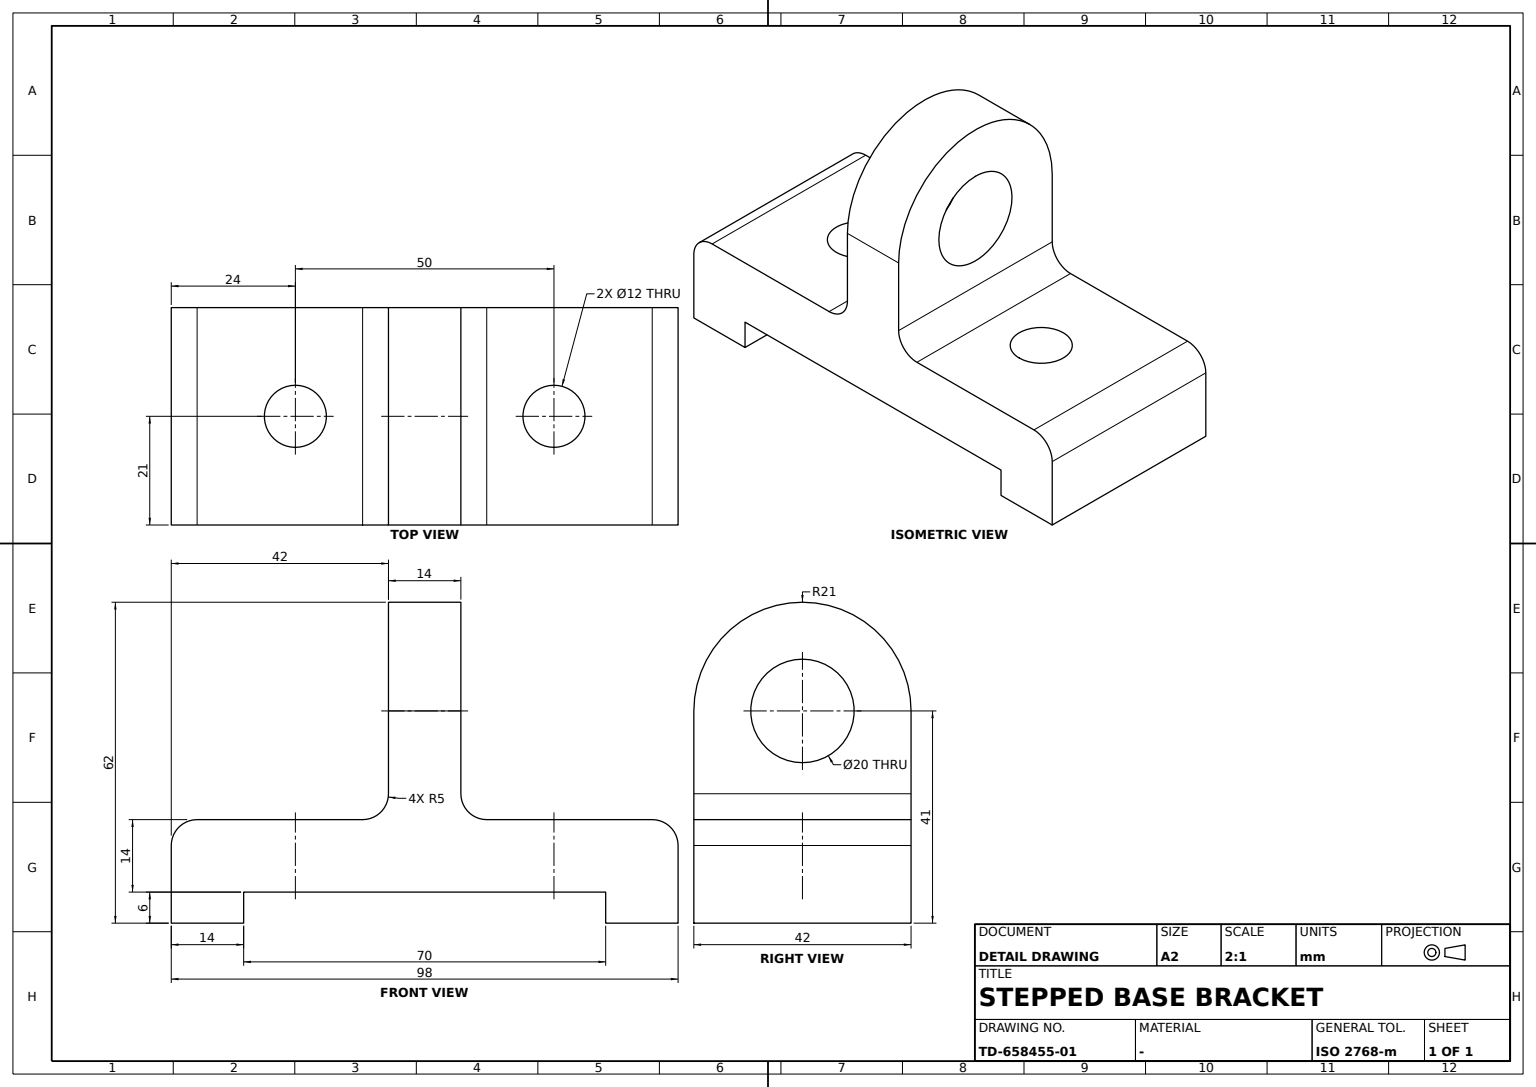
ISO-10303-21;
HEADER;
FILE_DESCRIPTION((''),'2;1');
FILE_NAME('','',(''),(''),'','','');
FILE_SCHEMA(('AUTOMOTIVE_DESIGN'));
ENDSEC;
DATA;
#1=APPLICATION_CONTEXT('');
#2=PRODUCT_CONTEXT('',#1,'mechanical');
#3=PRODUCT('','','',(#2));
#4=PRODUCT_DEFINITION_FORMATION('','',#3);
#5=PRODUCT_DEFINITION_CONTEXT('',#1,'design');
#6=PRODUCT_DEFINITION('','',#4,#5);
#7=PRODUCT_DEFINITION_SHAPE('','',#6);
#8=(LENGTH_UNIT()NAMED_UNIT(*)SI_UNIT(.MILLI.,.METRE.));
#9=(NAMED_UNIT(*)PLANE_ANGLE_UNIT()SI_UNIT($,.RADIAN.));
#10=(NAMED_UNIT(*)SI_UNIT($,.STERADIAN.)SOLID_ANGLE_UNIT());
#11=UNCERTAINTY_MEASURE_WITH_UNIT(LENGTH_MEASURE(0.005),#8,'distance_accuracy_value','');
#12=(GEOMETRIC_REPRESENTATION_CONTEXT(3)GLOBAL_UNCERTAINTY_ASSIGNED_CONTEXT((#11))GLOBAL_UNIT_ASSIGNED_CONTEXT((#8,#9,#10))REPRESENTATION_CONTEXT('',''));
#13=CARTESIAN_POINT('',(-21.,35.,-7.));
#14=VERTEX_POINT('',#13);
#15=CARTESIAN_POINT('',(-21.,35.,-13.));
#16=VERTEX_POINT('',#15);
#17=CARTESIAN_POINT('',(-21.,35.,0.));
#18=DIRECTION('',(0.,0.,-1.));
#19=VECTOR('',#18,1000.);
#20=LINE('',#17,#19);
#21=EDGE_CURVE('',#14,#16,#20,.T.);
#22=ORIENTED_EDGE('',*,*,#21,.T.);
#23=CARTESIAN_POINT('',(21.,35.,-13.));
#24=VERTEX_POINT('',#23);
#25=CARTESIAN_POINT('',(0.,35.,-13.));
#26=DIRECTION('',(1.,0.,0.));
#27=VECTOR('',#26,1000.);
#28=LINE('',#25,#27);
#29=EDGE_CURVE('',#16,#24,#28,.T.);
#30=ORIENTED_EDGE('',*,*,#29,.T.);
#31=CARTESIAN_POINT('',(21.,35.,-7.));
#32=VERTEX_POINT('',#31);
#33=CARTESIAN_POINT('',(21.,35.,0.));
#34=LINE('',#33,#19);
#35=EDGE_CURVE('',#32,#24,#34,.T.);
#36=ORIENTED_EDGE('',*,*,#35,.F.);
#37=CARTESIAN_POINT('',(0.,35.,-7.));
#38=LINE('',#37,#27);
#39=EDGE_CURVE('',#14,#32,#38,.T.);
#40=ORIENTED_EDGE('',*,*,#39,.F.);
#41=EDGE_LOOP('',(#22,#30,#36,#40));
#42=FACE_BOUND('',#41,.T.);
#43=DIRECTION('',(0.,-1.,0.));
#44=AXIS2_PLACEMENT_3D('',#37,#43,#18);
#45=PLANE('',#44);
#46=ADVANCED_FACE('',(#42),#45,.T.);
#47=CARTESIAN_POINT('',(21.,12.,7.));
#48=VERTEX_POINT('',#47);
#49=CARTESIAN_POINT('',(-21.,12.,7.));
#50=VERTEX_POINT('',#49);
#51=CARTESIAN_POINT('',(0.,12.,7.));
#52=DIRECTION('',(-1.,0.,0.));
#53=VECTOR('',#52,1000.);
#54=LINE('',#51,#53);
#55=EDGE_CURVE('',#48,#50,#54,.T.);
#56=ORIENTED_EDGE('',*,*,#55,.T.);
#57=CARTESIAN_POINT('',(-21.,7.,12.));
#58=VERTEX_POINT('',#57);
#59=CARTESIAN_POINT('',(-21.,12.,12.));
#60=AXIS2_PLACEMENT_3D('',#59,#26,#18);
#61=CIRCLE('',#60,5.);
#62=EDGE_CURVE('',#58,#50,#61,.T.);
#63=ORIENTED_EDGE('',*,*,#62,.F.);
#64=CARTESIAN_POINT('',(21.,7.,12.));
#65=VERTEX_POINT('',#64);
#66=CARTESIAN_POINT('',(0.,7.,12.));
#67=LINE('',#66,#53);
#68=EDGE_CURVE('',#65,#58,#67,.T.);
#69=ORIENTED_EDGE('',*,*,#68,.F.);
#70=CARTESIAN_POINT('',(21.,12.,12.));
#71=AXIS2_PLACEMENT_3D('',#70,#26,#18);
#72=CIRCLE('',#71,5.);
#73=EDGE_CURVE('',#65,#48,#72,.T.);
#74=ORIENTED_EDGE('',*,*,#73,.T.);
#75=EDGE_LOOP('',(#56,#63,#69,#74));
#76=FACE_BOUND('',#75,.T.);
#77=CARTESIAN_POINT('',(0.,12.,12.));
#78=AXIS2_PLACEMENT_3D('',#77,#52,#18);
#79=CYLINDRICAL_SURFACE('',#78,5.);
#80=ADVANCED_FACE('',(#76),#79,.F.);
#81=CARTESIAN_POINT('',(-21.,-35.,-7.));
#82=VERTEX_POINT('',#81);
#83=CARTESIAN_POINT('',(21.,-35.,-7.));
#84=VERTEX_POINT('',#83);
#85=CARTESIAN_POINT('',(0.,-35.,-7.));
#86=LINE('',#85,#27);
#87=EDGE_CURVE('',#82,#84,#86,.T.);
#88=ORIENTED_EDGE('',*,*,#87,.T.);
#89=CARTESIAN_POINT('',(21.,-35.,-13.));
#90=VERTEX_POINT('',#89);
#91=CARTESIAN_POINT('',(21.,-35.,0.));
#92=DIRECTION('',(0.,0.,1.));
#93=VECTOR('',#92,1000.);
#94=LINE('',#91,#93);
#95=EDGE_CURVE('',#90,#84,#94,.T.);
#96=ORIENTED_EDGE('',*,*,#95,.F.);
#97=CARTESIAN_POINT('',(-21.,-35.,-13.));
#98=VERTEX_POINT('',#97);
#99=CARTESIAN_POINT('',(0.,-35.,-13.));
#100=LINE('',#99,#27);
#101=EDGE_CURVE('',#98,#90,#100,.T.);
#102=ORIENTED_EDGE('',*,*,#101,.F.);
#103=CARTESIAN_POINT('',(-21.,-35.,0.));
#104=LINE('',#103,#93);
#105=EDGE_CURVE('',#98,#82,#104,.T.);
#106=ORIENTED_EDGE('',*,*,#105,.T.);
#107=EDGE_LOOP('',(#88,#96,#102,#106));
#108=FACE_BOUND('',#107,.T.);
#109=DIRECTION('',(0.,1.,0.));
#110=AXIS2_PLACEMENT_3D('',#99,#109,#92);
#111=PLANE('',#110);
#112=ADVANCED_FACE('',(#108),#111,.T.);
#113=CARTESIAN_POINT('',(-21.,49.,2.));
#114=VERTEX_POINT('',#113);
#115=CARTESIAN_POINT('',(21.,49.,2.));
#116=VERTEX_POINT('',#115);
#117=CARTESIAN_POINT('',(0.,49.,2.));
#118=LINE('',#117,#27);
#119=EDGE_CURVE('',#114,#116,#118,.T.);
#120=ORIENTED_EDGE('',*,*,#119,.F.);
#121=CARTESIAN_POINT('',(-21.,44.,7.));
#122=VERTEX_POINT('',#121);
#123=CARTESIAN_POINT('',(-21.,44.,2.));
#124=AXIS2_PLACEMENT_3D('',#123,#26,#18);
#125=CIRCLE('',#124,5.);
#126=EDGE_CURVE('',#114,#122,#125,.T.);
#127=ORIENTED_EDGE('',*,*,#126,.T.);
#128=CARTESIAN_POINT('',(21.,44.,7.));
#129=VERTEX_POINT('',#128);
#130=CARTESIAN_POINT('',(0.,44.,7.));
#131=LINE('',#130,#27);
#132=EDGE_CURVE('',#122,#129,#131,.T.);
#133=ORIENTED_EDGE('',*,*,#132,.T.);
#134=CARTESIAN_POINT('',(21.,44.,2.));
#135=AXIS2_PLACEMENT_3D('',#134,#26,#18);
#136=CIRCLE('',#135,5.);
#137=EDGE_CURVE('',#116,#129,#136,.T.);
#138=ORIENTED_EDGE('',*,*,#137,.F.);
#139=EDGE_LOOP('',(#120,#127,#133,#138));
#140=FACE_BOUND('',#139,.T.);
#141=CARTESIAN_POINT('',(0.,44.,2.));
#142=AXIS2_PLACEMENT_3D('',#141,#26,#92);
#143=CYLINDRICAL_SURFACE('',#142,5.);
#144=ADVANCED_FACE('',(#140),#143,.T.);
#145=CARTESIAN_POINT('',(-21.,-49.,-13.));
#146=VERTEX_POINT('',#145);
#147=CARTESIAN_POINT('',(-21.,0.,-13.));
#148=VECTOR('',#109,1000.);
#149=LINE('',#147,#148);
#150=EDGE_CURVE('',#146,#98,#149,.T.);
#151=ORIENTED_EDGE('',*,*,#150,.T.);
#152=ORIENTED_EDGE('',*,*,#101,.T.);
#153=CARTESIAN_POINT('',(21.,-49.,-13.));
#154=VERTEX_POINT('',#153);
#155=CARTESIAN_POINT('',(21.,0.,-13.));
#156=LINE('',#155,#148);
#157=EDGE_CURVE('',#154,#90,#156,.T.);
#158=ORIENTED_EDGE('',*,*,#157,.F.);
#159=CARTESIAN_POINT('',(0.,-49.,-13.));
#160=LINE('',#159,#27);
#161=EDGE_CURVE('',#146,#154,#160,.T.);
#162=ORIENTED_EDGE('',*,*,#161,.F.);
#163=EDGE_LOOP('',(#151,#152,#158,#162));
#164=FACE_BOUND('',#163,.T.);
#165=AXIS2_PLACEMENT_3D('',#159,#18,#109);
#166=PLANE('',#165);
#167=ADVANCED_FACE('',(#164),#166,.T.);
#168=CARTESIAN_POINT('',(21.,7.,28.));
#169=VERTEX_POINT('',#168);
#170=CARTESIAN_POINT('',(21.,7.,0.));
#171=LINE('',#170,#19);
#172=EDGE_CURVE('',#169,#65,#171,.T.);
#173=ORIENTED_EDGE('',*,*,#172,.T.);
#174=ORIENTED_EDGE('',*,*,#68,.T.);
#175=CARTESIAN_POINT('',(-21.,7.,28.));
#176=VERTEX_POINT('',#175);
#177=CARTESIAN_POINT('',(-21.,7.,0.));
#178=LINE('',#177,#19);
#179=EDGE_CURVE('',#176,#58,#178,.T.);
#180=ORIENTED_EDGE('',*,*,#179,.F.);
#181=CARTESIAN_POINT('',(0.,7.,28.));
#182=AXIS2_PLACEMENT_3D('',#181,#109,#92);
#183=CIRCLE('',#182,21.);
#184=EDGE_CURVE('',#176,#169,#183,.T.);
#185=ORIENTED_EDGE('',*,*,#184,.T.);
#186=EDGE_LOOP('',(#173,#174,#180,#185));
#187=FACE_BOUND('',#186,.T.);
#188=CARTESIAN_POINT('',(0.,7.,38.));
#189=VERTEX_POINT('',#188);
#190=CIRCLE('',#182,10.);
#191=EDGE_CURVE('',#189,#189,#190,.T.);
#192=ORIENTED_EDGE('',*,*,#191,.F.);
#193=EDGE_LOOP('',(#192));
#194=FACE_BOUND('',#193,.T.);
#195=CARTESIAN_POINT('',(0.,7.,0.));
#196=AXIS2_PLACEMENT_3D('',#195,#109,#52);
#197=PLANE('',#196);
#198=ADVANCED_FACE('',(#187,#194),#197,.T.);
#199=CARTESIAN_POINT('',(-6.,25.,-7.));
#200=VERTEX_POINT('',#199);
#201=CARTESIAN_POINT('',(0.,25.,-7.));
#202=AXIS2_PLACEMENT_3D('',#201,#18,#52);
#203=CIRCLE('',#202,6.);
#204=EDGE_CURVE('',#200,#200,#203,.T.);
#205=ORIENTED_EDGE('',*,*,#204,.T.);
#206=EDGE_LOOP('',(#205));
#207=FACE_BOUND('',#206,.T.);
#208=CARTESIAN_POINT('',(6.,25.,7.));
#209=VERTEX_POINT('',#208);
#210=CARTESIAN_POINT('',(0.,25.,7.));
#211=AXIS2_PLACEMENT_3D('',#210,#92,#26);
#212=CIRCLE('',#211,6.);
#213=EDGE_CURVE('',#209,#209,#212,.T.);
#214=ORIENTED_EDGE('',*,*,#213,.T.);
#215=EDGE_LOOP('',(#214));
#216=FACE_BOUND('',#215,.T.);
#217=CARTESIAN_POINT('',(0.,25.,-3.66));
#218=AXIS2_PLACEMENT_3D('',#217,#92,#109);
#219=CYLINDRICAL_SURFACE('',#218,6.);
#220=ADVANCED_FACE('',(#207,#216),#219,.F.);
#221=CARTESIAN_POINT('',(-6.,-25.,-7.));
#222=VERTEX_POINT('',#221);
#223=CARTESIAN_POINT('',(0.,-25.,-7.));
#224=AXIS2_PLACEMENT_3D('',#223,#18,#52);
#225=CIRCLE('',#224,6.);
#226=EDGE_CURVE('',#222,#222,#225,.T.);
#227=ORIENTED_EDGE('',*,*,#226,.F.);
#228=EDGE_LOOP('',(#227));
#229=FACE_BOUND('',#228,.T.);
#230=ORIENTED_EDGE('',*,*,#204,.F.);
#231=EDGE_LOOP('',(#230));
#232=FACE_BOUND('',#231,.T.);
#233=CARTESIAN_POINT('',(-21.,0.,-7.));
#234=LINE('',#233,#148);
#235=EDGE_CURVE('',#82,#14,#234,.T.);
#236=ORIENTED_EDGE('',*,*,#235,.T.);
#237=ORIENTED_EDGE('',*,*,#39,.T.);
#238=CARTESIAN_POINT('',(21.,0.,-7.));
#239=LINE('',#238,#148);
#240=EDGE_CURVE('',#84,#32,#239,.T.);
#241=ORIENTED_EDGE('',*,*,#240,.F.);
#242=ORIENTED_EDGE('',*,*,#87,.F.);
#243=EDGE_LOOP('',(#236,#237,#241,#242));
#244=FACE_BOUND('',#243,.T.);
#245=AXIS2_PLACEMENT_3D('',#85,#18,#109);
#246=PLANE('',#245);
#247=ADVANCED_FACE('',(#229,#232,#244),#246,.T.);
#248=CARTESIAN_POINT('',(-21.,-44.,7.));
#249=VERTEX_POINT('',#248);
#250=CARTESIAN_POINT('',(-21.,-49.,2.));
#251=VERTEX_POINT('',#250);
#252=CARTESIAN_POINT('',(-21.,-44.,2.));
#253=AXIS2_PLACEMENT_3D('',#252,#26,#18);
#254=CIRCLE('',#253,5.);
#255=EDGE_CURVE('',#249,#251,#254,.T.);
#256=ORIENTED_EDGE('',*,*,#255,.T.);
#257=CARTESIAN_POINT('',(21.,-49.,2.));
#258=VERTEX_POINT('',#257);
#259=CARTESIAN_POINT('',(0.,-49.,2.));
#260=LINE('',#259,#27);
#261=EDGE_CURVE('',#251,#258,#260,.T.);
#262=ORIENTED_EDGE('',*,*,#261,.T.);
#263=CARTESIAN_POINT('',(21.,-44.,7.));
#264=VERTEX_POINT('',#263);
#265=CARTESIAN_POINT('',(21.,-44.,2.));
#266=AXIS2_PLACEMENT_3D('',#265,#26,#18);
#267=CIRCLE('',#266,5.);
#268=EDGE_CURVE('',#264,#258,#267,.T.);
#269=ORIENTED_EDGE('',*,*,#268,.F.);
#270=CARTESIAN_POINT('',(0.,-44.,7.));
#271=LINE('',#270,#27);
#272=EDGE_CURVE('',#249,#264,#271,.T.);
#273=ORIENTED_EDGE('',*,*,#272,.F.);
#274=EDGE_LOOP('',(#256,#262,#269,#273));
#275=FACE_BOUND('',#274,.T.);
#276=CARTESIAN_POINT('',(0.,-44.,2.));
#277=AXIS2_PLACEMENT_3D('',#276,#26,#43);
#278=CYLINDRICAL_SURFACE('',#277,5.);
#279=ADVANCED_FACE('',(#275),#278,.T.);
#280=CARTESIAN_POINT('',(21.,49.,-13.));
#281=VERTEX_POINT('',#280);
#282=EDGE_CURVE('',#24,#281,#156,.T.);
#283=ORIENTED_EDGE('',*,*,#282,.T.);
#284=CARTESIAN_POINT('',(21.,49.,0.));
#285=LINE('',#284,#93);
#286=EDGE_CURVE('',#281,#116,#285,.T.);
#287=ORIENTED_EDGE('',*,*,#286,.T.);
#288=ORIENTED_EDGE('',*,*,#137,.T.);
#289=CARTESIAN_POINT('',(21.,0.,7.));
#290=VECTOR('',#43,1000.);
#291=LINE('',#289,#290);
#292=EDGE_CURVE('',#129,#48,#291,.T.);
#293=ORIENTED_EDGE('',*,*,#292,.T.);
#294=ORIENTED_EDGE('',*,*,#73,.F.);
#295=ORIENTED_EDGE('',*,*,#172,.F.);
#296=CARTESIAN_POINT('',(21.,-7.,28.));
#297=VERTEX_POINT('',#296);
#298=CARTESIAN_POINT('',(21.,0.,28.));
#299=LINE('',#298,#148);
#300=EDGE_CURVE('',#297,#169,#299,.T.);
#301=ORIENTED_EDGE('',*,*,#300,.F.);
#302=CARTESIAN_POINT('',(21.,-7.,12.));
#303=VERTEX_POINT('',#302);
#304=CARTESIAN_POINT('',(21.,-7.,0.));
#305=LINE('',#304,#19);
#306=EDGE_CURVE('',#297,#303,#305,.T.);
#307=ORIENTED_EDGE('',*,*,#306,.T.);
#308=CARTESIAN_POINT('',(21.,-12.,7.));
#309=VERTEX_POINT('',#308);
#310=CARTESIAN_POINT('',(21.,-12.,12.));
#311=AXIS2_PLACEMENT_3D('',#310,#26,#18);
#312=CIRCLE('',#311,5.);
#313=EDGE_CURVE('',#309,#303,#312,.T.);
#314=ORIENTED_EDGE('',*,*,#313,.F.);
#315=EDGE_CURVE('',#309,#264,#291,.T.);
#316=ORIENTED_EDGE('',*,*,#315,.T.);
#317=ORIENTED_EDGE('',*,*,#268,.T.);
#318=CARTESIAN_POINT('',(21.,-49.,0.));
#319=LINE('',#318,#19);
#320=EDGE_CURVE('',#258,#154,#319,.T.);
#321=ORIENTED_EDGE('',*,*,#320,.T.);
#322=ORIENTED_EDGE('',*,*,#157,.T.);
#323=ORIENTED_EDGE('',*,*,#95,.T.);
#324=ORIENTED_EDGE('',*,*,#240,.T.);
#325=ORIENTED_EDGE('',*,*,#35,.T.);
#326=EDGE_LOOP('',(#283,#287,#288,#293,#294,#295,#301,#307,#314,#316,#317,#321,#322,#323,#324,#325));
#327=FACE_BOUND('',#326,.T.);
#328=CARTESIAN_POINT('',(21.,0.,0.));
#329=AXIS2_PLACEMENT_3D('',#328,#26,#109);
#330=PLANE('',#329);
#331=ADVANCED_FACE('',(#327),#330,.T.);
#332=ORIENTED_EDGE('',*,*,#306,.F.);
#333=CARTESIAN_POINT('',(-21.,-7.,28.));
#334=VERTEX_POINT('',#333);
#335=CARTESIAN_POINT('',(0.,-7.,28.));
#336=AXIS2_PLACEMENT_3D('',#335,#109,#92);
#337=CIRCLE('',#336,21.);
#338=EDGE_CURVE('',#334,#297,#337,.T.);
#339=ORIENTED_EDGE('',*,*,#338,.F.);
#340=CARTESIAN_POINT('',(-21.,-7.,12.));
#341=VERTEX_POINT('',#340);
#342=CARTESIAN_POINT('',(-21.,-7.,0.));
#343=LINE('',#342,#19);
#344=EDGE_CURVE('',#334,#341,#343,.T.);
#345=ORIENTED_EDGE('',*,*,#344,.T.);
#346=CARTESIAN_POINT('',(0.,-7.,12.));
#347=LINE('',#346,#27);
#348=EDGE_CURVE('',#341,#303,#347,.T.);
#349=ORIENTED_EDGE('',*,*,#348,.T.);
#350=EDGE_LOOP('',(#332,#339,#345,#349));
#351=FACE_BOUND('',#350,.T.);
#352=CARTESIAN_POINT('',(0.,-7.,38.));
#353=VERTEX_POINT('',#352);
#354=CIRCLE('',#336,10.);
#355=EDGE_CURVE('',#353,#353,#354,.T.);
#356=ORIENTED_EDGE('',*,*,#355,.T.);
#357=EDGE_LOOP('',(#356));
#358=FACE_BOUND('',#357,.T.);
#359=CARTESIAN_POINT('',(0.,-7.,0.));
#360=AXIS2_PLACEMENT_3D('',#359,#109,#52);
#361=PLANE('',#360);
#362=ADVANCED_FACE('',(#351,#358),#361,.F.);
#363=CARTESIAN_POINT('',(-21.,49.,-13.));
#364=VERTEX_POINT('',#363);
#365=EDGE_CURVE('',#16,#364,#149,.T.);
#366=ORIENTED_EDGE('',*,*,#365,.T.);
#367=CARTESIAN_POINT('',(0.,49.,-13.));
#368=LINE('',#367,#27);
#369=EDGE_CURVE('',#364,#281,#368,.T.);
#370=ORIENTED_EDGE('',*,*,#369,.T.);
#371=ORIENTED_EDGE('',*,*,#282,.F.);
#372=ORIENTED_EDGE('',*,*,#29,.F.);
#373=EDGE_LOOP('',(#366,#370,#371,#372));
#374=FACE_BOUND('',#373,.T.);
#375=ADVANCED_FACE('',(#374),#166,.T.);
#376=ORIENTED_EDGE('',*,*,#338,.T.);
#377=ORIENTED_EDGE('',*,*,#300,.T.);
#378=ORIENTED_EDGE('',*,*,#184,.F.);
#379=CARTESIAN_POINT('',(-21.,0.,28.));
#380=LINE('',#379,#148);
#381=EDGE_CURVE('',#334,#176,#380,.T.);
#382=ORIENTED_EDGE('',*,*,#381,.F.);
#383=EDGE_LOOP('',(#376,#377,#378,#382));
#384=FACE_BOUND('',#383,.T.);
#385=CARTESIAN_POINT('',(0.,0.,28.));
#386=AXIS2_PLACEMENT_3D('',#385,#109,#52);
#387=CYLINDRICAL_SURFACE('',#386,21.);
#388=ADVANCED_FACE('',(#384),#387,.T.);
#389=ORIENTED_EDGE('',*,*,#369,.F.);
#390=CARTESIAN_POINT('',(-21.,49.,0.));
#391=LINE('',#390,#93);
#392=EDGE_CURVE('',#364,#114,#391,.T.);
#393=ORIENTED_EDGE('',*,*,#392,.T.);
#394=ORIENTED_EDGE('',*,*,#119,.T.);
#395=ORIENTED_EDGE('',*,*,#286,.F.);
#396=EDGE_LOOP('',(#389,#393,#394,#395));
#397=FACE_BOUND('',#396,.T.);
#398=AXIS2_PLACEMENT_3D('',#367,#109,#92);
#399=PLANE('',#398);
#400=ADVANCED_FACE('',(#397),#399,.T.);
#401=ORIENTED_EDGE('',*,*,#292,.F.);
#402=ORIENTED_EDGE('',*,*,#132,.F.);
#403=CARTESIAN_POINT('',(-21.,0.,7.));
#404=LINE('',#403,#290);
#405=EDGE_CURVE('',#122,#50,#404,.T.);
#406=ORIENTED_EDGE('',*,*,#405,.T.);
#407=ORIENTED_EDGE('',*,*,#55,.F.);
#408=EDGE_LOOP('',(#401,#402,#406,#407));
#409=FACE_BOUND('',#408,.T.);
#410=ORIENTED_EDGE('',*,*,#213,.F.);
#411=EDGE_LOOP('',(#410));
#412=FACE_BOUND('',#411,.T.);
#413=CARTESIAN_POINT('',(0.,49.,7.));
#414=AXIS2_PLACEMENT_3D('',#413,#92,#43);
#415=PLANE('',#414);
#416=ADVANCED_FACE('',(#409,#412),#415,.T.);
#417=ORIENTED_EDGE('',*,*,#365,.F.);
#418=ORIENTED_EDGE('',*,*,#21,.F.);
#419=ORIENTED_EDGE('',*,*,#235,.F.);
#420=ORIENTED_EDGE('',*,*,#105,.F.);
#421=ORIENTED_EDGE('',*,*,#150,.F.);
#422=CARTESIAN_POINT('',(-21.,-49.,0.));
#423=LINE('',#422,#19);
#424=EDGE_CURVE('',#251,#146,#423,.T.);
#425=ORIENTED_EDGE('',*,*,#424,.F.);
#426=ORIENTED_EDGE('',*,*,#255,.F.);
#427=CARTESIAN_POINT('',(-21.,-12.,7.));
#428=VERTEX_POINT('',#427);
#429=EDGE_CURVE('',#428,#249,#404,.T.);
#430=ORIENTED_EDGE('',*,*,#429,.F.);
#431=CARTESIAN_POINT('',(-21.,-12.,12.));
#432=AXIS2_PLACEMENT_3D('',#431,#26,#18);
#433=CIRCLE('',#432,5.);
#434=EDGE_CURVE('',#428,#341,#433,.T.);
#435=ORIENTED_EDGE('',*,*,#434,.T.);
#436=ORIENTED_EDGE('',*,*,#344,.F.);
#437=ORIENTED_EDGE('',*,*,#381,.T.);
#438=ORIENTED_EDGE('',*,*,#179,.T.);
#439=ORIENTED_EDGE('',*,*,#62,.T.);
#440=ORIENTED_EDGE('',*,*,#405,.F.);
#441=ORIENTED_EDGE('',*,*,#126,.F.);
#442=ORIENTED_EDGE('',*,*,#392,.F.);
#443=EDGE_LOOP('',(#417,#418,#419,#420,#421,#425,#426,#430,#435,#436,#437,#438,#439,#440,#441,#442));
#444=FACE_BOUND('',#443,.T.);
#445=CARTESIAN_POINT('',(-21.,0.,0.));
#446=AXIS2_PLACEMENT_3D('',#445,#26,#109);
#447=PLANE('',#446);
#448=ADVANCED_FACE('',(#444),#447,.F.);
#449=ORIENTED_EDGE('',*,*,#355,.F.);
#450=EDGE_LOOP('',(#449));
#451=FACE_BOUND('',#450,.T.);
#452=ORIENTED_EDGE('',*,*,#191,.T.);
#453=EDGE_LOOP('',(#452));
#454=FACE_BOUND('',#453,.T.);
#455=CYLINDRICAL_SURFACE('',#386,10.);
#456=ADVANCED_FACE('',(#451,#454),#455,.F.);
#457=CARTESIAN_POINT('',(6.,-25.,7.));
#458=VERTEX_POINT('',#457);
#459=CARTESIAN_POINT('',(0.,-25.,7.));
#460=AXIS2_PLACEMENT_3D('',#459,#92,#26);
#461=CIRCLE('',#460,6.);
#462=EDGE_CURVE('',#458,#458,#461,.T.);
#463=ORIENTED_EDGE('',*,*,#462,.T.);
#464=EDGE_LOOP('',(#463));
#465=FACE_BOUND('',#464,.T.);
#466=ORIENTED_EDGE('',*,*,#226,.T.);
#467=EDGE_LOOP('',(#466));
#468=FACE_BOUND('',#467,.T.);
#469=CARTESIAN_POINT('',(0.,-25.,-3.66));
#470=AXIS2_PLACEMENT_3D('',#469,#92,#109);
#471=CYLINDRICAL_SURFACE('',#470,6.);
#472=ADVANCED_FACE('',(#465,#468),#471,.F.);
#473=ORIENTED_EDGE('',*,*,#315,.F.);
#474=CARTESIAN_POINT('',(0.,-12.,7.));
#475=LINE('',#474,#27);
#476=EDGE_CURVE('',#428,#309,#475,.T.);
#477=ORIENTED_EDGE('',*,*,#476,.F.);
#478=ORIENTED_EDGE('',*,*,#429,.T.);
#479=ORIENTED_EDGE('',*,*,#272,.T.);
#480=EDGE_LOOP('',(#473,#477,#478,#479));
#481=FACE_BOUND('',#480,.T.);
#482=ORIENTED_EDGE('',*,*,#462,.F.);
#483=EDGE_LOOP('',(#482));
#484=FACE_BOUND('',#483,.T.);
#485=ADVANCED_FACE('',(#481,#484),#415,.T.);
#486=ORIENTED_EDGE('',*,*,#424,.T.);
#487=ORIENTED_EDGE('',*,*,#161,.T.);
#488=ORIENTED_EDGE('',*,*,#320,.F.);
#489=ORIENTED_EDGE('',*,*,#261,.F.);
#490=EDGE_LOOP('',(#486,#487,#488,#489));
#491=FACE_BOUND('',#490,.T.);
#492=CARTESIAN_POINT('',(0.,-49.,7.));
#493=AXIS2_PLACEMENT_3D('',#492,#43,#18);
#494=PLANE('',#493);
#495=ADVANCED_FACE('',(#491),#494,.T.);
#496=ORIENTED_EDGE('',*,*,#313,.T.);
#497=ORIENTED_EDGE('',*,*,#348,.F.);
#498=ORIENTED_EDGE('',*,*,#434,.F.);
#499=ORIENTED_EDGE('',*,*,#476,.T.);
#500=EDGE_LOOP('',(#496,#497,#498,#499));
#501=FACE_BOUND('',#500,.T.);
#502=CARTESIAN_POINT('',(0.,-12.,12.));
#503=AXIS2_PLACEMENT_3D('',#502,#26,#109);
#504=CYLINDRICAL_SURFACE('',#503,5.);
#505=ADVANCED_FACE('',(#501),#504,.F.);
#506=CLOSED_SHELL('',(#46,#80,#112,#144,#167,#198,#220,#247,#279,#331,#362,#375,#388,#400,#416,#448,#456,#472,#485,#495,#505));
#507=MANIFOLD_SOLID_BREP('',#506);
#508=ADVANCED_BREP_SHAPE_REPRESENTATION('',(#507),#12);
#509=SHAPE_DEFINITION_REPRESENTATION(#7,#508);
ENDSEC;
END-ISO-10303-21;
